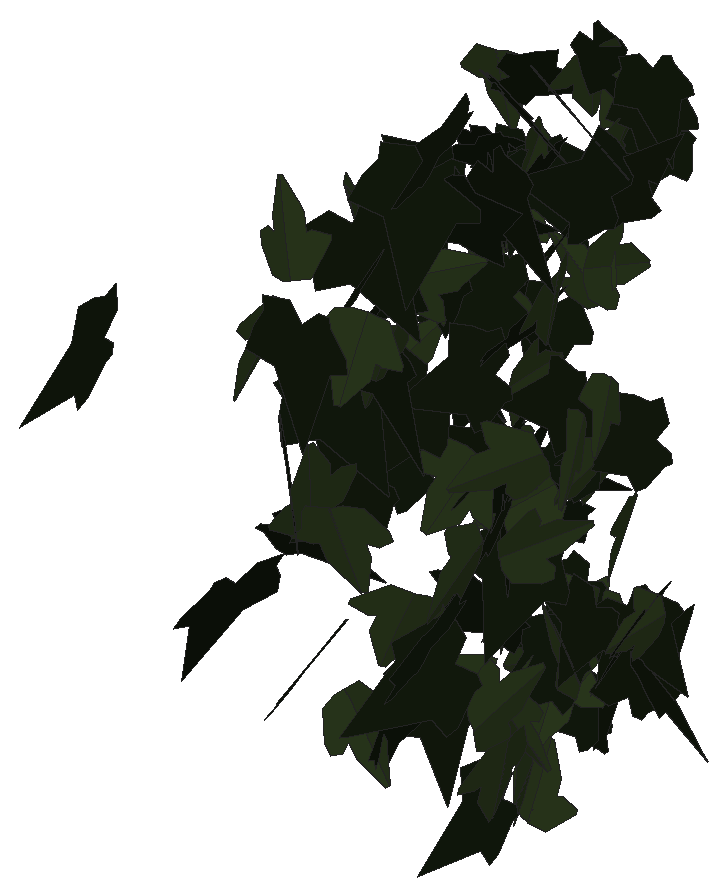
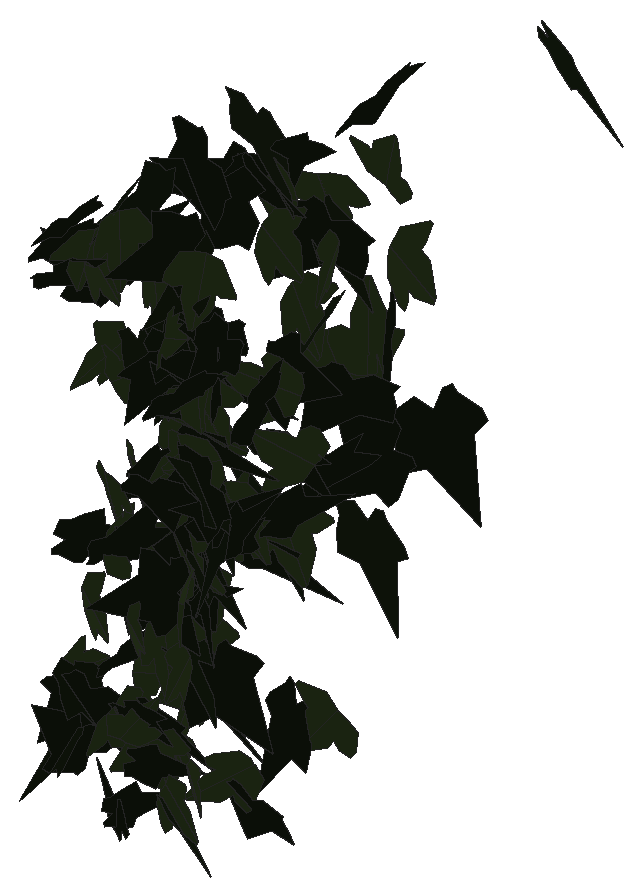
# SketchUp Ruby script. Lengths in inches.
U = 1.inch
M = Sketchup.active_model
def pt(a) = Geom::Point3d.new(a.map { |v| v * U })
def face(e, loops, mat)
  f = e.add_face(loops[0].map { |a| pt(a) })
  loops[1..].each { |l| e.add_face(l.map { |a| pt(a) }).erase! }
  f.material = f.back_material = mat if mat
  f
end
# faces: each face lists its corners as indices into pts; further lists are holes
def faces(e, pts, list, mat = nil) = list.each { |f| face(e, (f[0].is_a?(Array) ? f : [f]).map { |l| l.map { |i| pts[i] } }, mat) }
# xy, xz, yz: faces in a plane at the given z, y or x. An outline is a flat list of corners, or four numbers for a rectangle; further outlines are holes
def ring(l) = l.size == 4 ? [[l[0], l[1]], [l[2], l[1]], [l[2], l[3]], [l[0], l[3]]] : l.each_slice(2).to_a
def flat(e, list, mat, &to3) = list.each { |f| face(e, (f[0].is_a?(Array) ? f : [f]).map { |l| ring(l).map { |u, v| to3.(u, v) } }, mat) }
def xy(e, z, list, mat = nil) = flat(e, list, mat) { |x, y| [x, y, z] }
def xz(e, y, list, mat = nil) = flat(e, list, mat) { |x, z| [x, y, z] }
def yz(e, x, list, mat = nil) = flat(e, list, mat) { |y, z| [x, y, z] }
def lines(e, pts, list) = list.each { |a, b| e.add_line(pt(pts[a]), pt(pts[b])) }
# prism: a flat outline (further loops are holes) pulled along v
def prism(e, loops, v, mat = nil)
  f = face(e, loops, mat); d = Geom::Vector3d.new(v.map { |x| x * U })
  f.pushpull(f.normal.samedirection?(d) ? d.length : -d.length)
end
def box(e, o, s, mat = nil) = prism(e, [[o, [o[0] + s[0], o[1], o[2]], [o[0] + s[0], o[1] + s[1], o[2]], [o[0], o[1] + s[1], o[2]]]], [0, 0, s[2]], mat)
def at(x, y, z, deg = 0) = Geom::Transformation.translation(pt([x, y, z])) * Geom::Transformation.rotation(ORIGIN, Z_AXIS, deg.degrees)
def axes(o, x, y, z) = Geom::Transformation.new([*x, 0, *y, 0, *z, 0, *pt(o).to_a, 1])
def part(name) = M.definitions.add(name)
# library, detail: a bought-in or finely detailed component or shape, given as its bounding box
def library(name, o, s) = part(name).tap { |d| box(d.entities, o, s) }
def detail(e, o, s) = box(e.add_group.entities, o, s)
def put(e, d, t, mat = nil) = e.add_instance(d, t).tap { |i| i.material = mat if mat }
def group(e, t, mat = nil) = e.add_group.tap { |g| g.transformation = t; g.material = mat if mat }.entities
root = M.entities
M.materials.add("efeu1").color = [18, 25, 13]
M.materials.add("efeu2").color = [43, 57, 29]
c1 = part("ivyleaf_9")
p = [[1.54,2.16,1.25],[1.36,2.04,1.19],[-0.21,0.99,0.68],[-0.71,1.11,0.82],[-0.85,0.86,0.67],[-0.8,0.17,0.21],
  [-0.9,-0.01,0.1],[-0.67,-0.16,-0.02],[-0.08,-0.08,-0.05],[-0.03,-0.6,-0.4],[0.65,-0.88,-0.66],[0.83,-0.6,-0.49],
  [1.29,-0.42,-0.43],[1.8125,-0.07,-0.26],[1.21,0.44,0.15]]
faces(c1.entities,p,[[0,1,2,3,4,5,6,7,8,9,10,11,12,13,14]],"efeu1")
c2 = part("ivyleaf_10")
p = [[0,0.5,-0.03],[-0.0625,2.02,-0.43],[-0.19,2.01,-0.46],[-0.54,1.05,-0.29],[-0.52,0.625,-0.18],[-0.83,0.76,-0.28],
  [-1.16,0.64,-0.33],[-1.15,0.33,-0.24],[-0.77,-0.39,0.02],[-0.3,-0.51,0.16],[0.04,-0.48,0.23],[-0.02,2.01,-0.4375],
  [-0.06,2.01,-0.43],[0.04,-0.49,0.23],[0.67,-0.49,0.14],[1.38,0.36,-0.2],[1.375,0.51,-0.24],[0.81,0.65,-0.19],
  [0.62,0.59,-0.15],[0.6,1.09,-0.28],[0.5,1.23,-0.31]]
faces(c2.entities,p,[[0,1,2,3,4,5,6,7,8,9,10],[11,12,0,13,14,15,16,17,18,19,20]],"efeu2")
put(root,c1,axes([594.9,111.1,205.24],[-1.20311,0.67443,-0.22377],[0.18999,-0.11868,-1.37921],[-0.68471,-1.21797,0.01049]))
put(root,c1,axes([598.09,116.25,204.45],[0.0745,-1.25549,0.12259],[0.01675,-0.12181,-1.25766],[1.26135,0.07578,0.00946]))
put(root,c1,axes([594.7,117.4375,194.38],[-0.30601,1.14013,-0.69859],[0.15547,-0.68145,-1.18026],[-1.32807,-0.34248,0.0228]))
put(root,c2,axes([596.25,119.11,196.8125],[-0.28548,-1.16466,-0.34594],[-0.08339,-0.33574,1.19914],[-1.21208,0.29741,-0.00102]))
put(root,c1,axes([594.87,119.52,197.96],[0.12828,-0.08477,-1.23247],[1.18885,-0.3284,0.14633],[-0.33586,-1.19482,0.04722]))
put(root,c2,axes([597.12,119.09,196.59],[-1.14088,-0.33532,-0.23766],[0.23576,0.04044,-1.18883],[0.33666,-1.16467,0.02715]))
put(root,c2,axes([597.57,119.52,202.76],[1.09698,0.24304,-0.16363],[-0.15952,-0.03646,-1.12358],[-0.24576,1.10852,-0.00108]))
put(root,c2,axes([593.89,120.15,201.63],[0.2666,-0.99216,0.69498],[0.16277,-0.67582,-1.02724],[1.20037,0.312,-0.01506]))
put(root,c2,axes([594.92,119.72,204.11],[1.07624,-0.08575,0.44382],[-0.43931,0.07148,1.07913],[-0.10645,-1.16196,0.03363]))
put(root,c1,axes([595.5,119.875,191.06],[-0.49456,1.21146,0.07928],[-0.03156,0.07275,-1.30852],[-1.21364,-0.49556,0.00172]))
put(root,c1,axes([594.05,120.63,194.66],[1.08809,0.26212,0.32005],[0.31075,0.0766,-1.11922],[-0.27308,1.1316,0.00162]))
put(root,c1,axes([596.14,121.25,202.8],[-0.74032,0.84807,-0.33833],[0.22298,-0.25445,-1.12574],[-0.88542,-0.77317,-0.00062]))
put(root,c1,axes([598.46,121.56,191.92],[-0.60702,1.1525,0.22615],[-0.15966,0.17124,-1.30117],[-1.16357,-0.62474,0.06056]))
put(root,c1,axes([598.18,122.84,190.66],[-1.26764,-0.15024,0.27481],[-0.26251,-0.11522,-1.27389],[0.17082,-1.29195,0.08166]))
put(root,c2,axes([596.03,122.76,200.54],[-0.0207,-1.07947,0.24208],[-0.01252,-0.24187,-1.07964],[1.1062,-0.02294,-0.00769]))
put(root,c2,axes([596.7,122.82,192.1],[-0.77403,-0.71989,0.40358],[-0.28667,-0.28432,-1.05698],[0.77391,-0.82532,0.01211]))
put(root,c1,axes([594.84,122.74,203.73],[-0.33428,-0.44901,-1.13368],[0.79121,0.81456,-0.55592],[0.9278,-0.85642,0.06562]))
put(root,c1,axes([596.86,123.4375,205.82],[-0.50897,-1.17452,-0.21721],[0.05931,0.21096,-1.27973],[1.19297,-0.51159,-0.02905]))
put(root,c1,axes([594.5,123.87,194.94],[-0.45546,-0.7442,0.79182],[-0.36336,-0.70483,-0.87145],[1.0241,-0.58106,0.04295]))
put(root,c1,axes([593.81,122.88,198.29],[-0.2402,-0.7174,-0.98343],[0.52576,0.84293,-0.74333],[1.09789,-0.56061,0.14081]))
put(root,c1,axes([595.05,123.26,199.78],[0.70864,-1.15375,-0.04659],[-0.01528,0.04529,-1.35395],[1.15458,0.70872,0.01068]))
put(root,c1,axes([597.48,123.1,206.84],[-0.53357,1.12789,0.44328],[-0.27597,0.35853,-1.24444],[-1.18003,-0.59384,0.09059]))
put(root,c2,axes([595.58,124.06,204.99],[-0.32373,0.31033,-1.05872],[0.8146,-0.67688,-0.44749],[-0.74406,-0.87608,-0.02929]))
put(root,c2,axes([599.0625,124.15,187.55],[0.00145,-1.23722,-0.02442],[0.0218,0.02444,-1.23703],[1.23727,0.00102,0.02182]))
put(root,c2,axes([597.16,124.94,192.93],[0.12007,-0.39198,1.14556],[0.44623,-1.05582,-0.40804],[1.12554,0.4604,0.03957]))
put(root,c1,axes([596.91,123.91,205.14],[-0.72385,-0.02588,-0.87365],[-0.87227,-0.05072,0.72421],[-0.05556,1.13343,0.01246]))
put(root,c2,axes([593.65,124.12,203.65],[-0.7185,0.75396,-0.07109],[0.04465,-0.05565,-1.04148],[-0.75599,-0.71987,0.00605]))
put(root,c1,axes([598.65,124.46,185.74],[-1.17691,0.31113,-0.06093],[0.05753,-0.0208,-1.21733],[-0.31177,-1.1783,0.0054]))
put(root,c1,axes([597.14,124.28,204.4375],[0.75648,0.33779,-0.92743],[0.76873,0.53128,0.82054],[0.6191,-1.07244,0.11438]))
put(root,c2,axes([593.26,124.52,186.78],[0.85944,0.05689,0.79181],[0.78275,0.13373,-0.85922],[-0.13229,1.16091,0.06018]))
put(root,c1,axes([598.35,124.74,205.71],[-0.18682,-0.06636,-1.28296],[1.23249,0.35651,-0.19791],[0.36245,-1.24651,0.01169]))
put(root,c2,axes([598.74,123.77,188.82],[0.07731,0.27266,-1.16452],[0.37166,1.1037,0.28309],[1.13681,-0.37938,-0.01336]))
put(root,c2,axes([594.9,125.6,204.46],[0.07768,-0.94291,0.60554],[0.09727,-0.59903,-0.94525],[1.11638,0.1178,0.04023]))
put(root,c2,axes([598.57,125.69,196.26],[-0.2748,-0.36508,1.04422],[-0.64122,-0.82417,-0.45689],[0.90139,-0.69759,-0.00668]))
put(root,c1,axes([594.84,125.72,197],[-1.18345,-0.33009,-0.14086],[0.14235,0.01385,-1.22838],[0.32945,-1.19173,0.02474]))
put(root,c1,axes([597.35,125.73,198.55],[-0.96344,0.00137,0.49421],[-0.49418,0.00887,-0.96341],[-0.00527,-1.08276,-0.00727]))
put(root,c1,axes([594.375,126.14,194.43],[-0.43172,-0.27867,0.83565],[-0.63499,-0.54656,-0.51031],[0.61054,-0.76549,0.06015]))
put(root,c1,axes([594.01,126.54,200.28],[-0.50797,0.10068,-0.93521],[0.47648,-0.88887,-0.3545],[-0.81101,-0.58529,0.3775]))
put(root,c1,axes([594.47,124.98,186.88],[-0.14259,0.12416,-1.22895],[-0.85525,0.88268,0.18841],[0.89122,0.86691,-0.01583]))
put(root,c2,axes([597.86,126.67,185.43],[-0.04899,0.07828,1.13161],[0.76419,-0.83476,0.09083],[0.83826,0.76558,-0.01667]))
put(root,c2,axes([596,126.24,194.73],[1.11903,-0.15908,-0.48461],[-0.4793,0.07159,-1.13028],[0.17442,1.21736,0.00314]))
put(root,c2,axes([599.24,126.19,201.95],[0.22876,-1.14299,-0.23813],[-0.03512,0.23581,-1.1656],[1.167,0.23115,0.0116]))
put(root,c2,axes([597.5,126.34,187.57],[-0.71977,0.24817,-0.71613],[0.66548,-0.26573,-0.76094],[-0.36273,-0.97995,0.02498]))
put(root,c2,axes([593.23,126.08,197.03],[0.47905,0.46185,-0.89118],[0.64311,0.61694,0.66542],[0.77066,-0.80192,-0.00133]))
put(root,c2,axes([598.19,126.7,184.47],[1.00415,-0.13155,-0.12814],[0.12988,0.00515,1.0125],[-0.12983,-1.01228,0.0218]))
put(root,c1,axes([596.81,126.48,195.22],[-0.41451,1.0853,0.27622],[-0.14478,0.24013,-1.16076],[-1.1105,-0.4364,0.04823]))
put(root,c1,axes([597.64,126.23,199.7],[0.25674,0.98822,0.60672],[0.05834,0.60962,-1.01763],[-1.15814,0.24978,0.08324]))
put(root,c1,axes([596.46,127.47,193.17],[-0.85719,0.52427,-0.63273],[0.52037,-0.36129,-1.00433],[-0.63594,-1.00229,0.03106]))
put(root,c2,axes([593.42,126.91,199.89],[0.33092,0.06052,-1.1124],[1.08765,0.23357,0.33627],[0.24108,-1.13683,0.00987]))
put(root,c2,axes([597.75,126.57,192.53],[0.07707,-0.32794,1.07701],[0.26087,1.05535,0.30268],[-1.09519,0.22831,0.14789]))
put(root,c1,axes([595.4,127.75,194.13],[0.13124,0.00441,0.93921],[-0.90052,-0.26881,0.1271],[0.26681,-0.90944,-0.03301]))
put(root,c1,axes([593.59,128.3,199.82],[0.23887,-0.51465,-1.0461],[0.55581,-0.88839,0.56399],[-1.02482,-0.60177,0.06204]))
put(root,c1,axes([596.72,128.18,191.48],[-0.58311,-1.01327,0.05954],[0.0237,-0.08224,-1.16746],[1.01475,-0.58034,0.06148]))
put(root,c1,axes([596.42,127.47,192.54],[0.1951,-0.0134,-1.18093],[-1.17095,0.15371,-0.19519],[0.15383,1.18703,0.01194]))
put(root,c2,axes([598.39,128.28,195.9],[0.88414,-0.70101,0.1802],[0.14546,-0.10659,-1.1283],[0.70904,0.896,0.00677]))
put(root,c1,axes([599.05,128.9,203.59],[-0.13514,-0.10869,1.14619],[-0.86731,-0.74937,-0.17332],[0.75719,-0.87776,0.00605]))
put(root,c2,axes([596.95,128.33,193.45],[0.73138,0.04132,-0.84086],[-0.83782,-0.07346,-0.73235],[-0.08253,1.11201,-0.01714]))
put(root,c1,axes([595.26,128.1,189.43],[0.06919,0.53824,-1.02259],[-0.86814,-0.65192,-0.40188],[-0.7627,0.79087,0.36467]))
put(root,c1,axes([593.3,128.62,185.47],[-0.60254,-0.44485,-0.79269],[0.79197,0.20986,-0.71976],[0.44614,-0.97333,0.20711]))
put(root,c1,axes([596.26,127.46,193.14],[0.08916,0.08245,1.19053],[0.4124,1.11817,-0.10832],[-1.11986,0.41834,0.05489]))
put(root,c1,axes([596.62,127.98,190.29],[-0.5249,1.0271,0.21942],[-0.11604,0.18708,-1.15332],[-1.04385,-0.53727,0.01787]))
put(root,c1,axes([597.55,129.27,196.27],[0.05233,-0.73378,-0.62109],[0.15857,-0.60691,0.73038],[-0.94818,-0.14199,0.08786]))
put(root,c2,axes([598.28,128.1,188.27],[-0.30993,0.35557,-0.99241],[-0.70903,0.69518,0.47051],[0.78013,0.77309,0.03336]))
put(root,c1,axes([598.16,129.4,189.58],[-0.24689,-0.83209,0.37404],[-0.06986,-0.36911,-0.86724],[0.90962,-0.25419,0.03491]))
put(root,c1,axes([593.74,129.49,195.25],[-0.12385,-0.18483,0.88129],[-0.48049,-0.73878,-0.22247],[0.76155,-0.49619,0.00296]))
put(root,c2,axes([593.94,128.44,186.23],[-0.39005,-0.289,-0.83354],[0.74463,0.38091,-0.48051],[0.47312,-0.83776,0.06907]))
put(root,c1,axes([597.03,128.96,206.24],[0.91232,-0.61368,0.33504],[0.29202,-0.16602,-1.09925],[0.63529,0.95761,0.02413]))
put(root,c2,axes([595.38,129.4375,193.61],[-0.03839,-0.0636,-0.9919],[0.66321,-0.74099,0.02184],[-0.74031,-0.66051,0.071]))
put(root,c1,axes([597.15,129.39,187.81],[-1.1226,0.03762,0.0796],[-0.08039,-0.02268,-1.12295],[-0.03591,-1.12519,0.0253]))
put(root,c2,axes([596.39,128.38,196.81],[0.08525,-0.0547,0.92635],[-0.24421,0.89614,0.07539],[-0.89525,-0.24966,0.06764]))
put(root,c1,axes([596.7,129.43,192.39],[0.08789,0.45969,-0.76832],[-0.18811,-0.7453,-0.46744],[-0.87535,0.20631,0.02331]))
put(root,c1,axes([594.95,129.56,198.56],[-0.8881,0.06353,0.49285],[-0.49544,-0.035,-0.88825],[-0.0385,-1.01509,0.06147]))
put(root,c2,axes([597.7,130.18,194.02],[-0.00668,-0.17973,1.03263],[0.27265,-0.9974,-0.17184],[1.01208,0.26751,0.0531]))
put(root,c2,axes([596.57,129.72,186.79],[0.73709,0.75243,-0.3262],[-0.20901,-0.25176,-1.05299],[-0.79302,0.76572,-0.02566]))
put(root,c2,axes([596.04,129.65,191.29],[-0.18669,-1.12325,-0.10035],[0.02217,0.09804,-1.13865],[1.12751,-0.18791,0.00577]))
put(root,c1,axes([598.72,129.3,203.11],[-0.19393,-0.11076,1.00396],[0.99024,0.18065,0.21121],[-0.19909,1.00643,0.07258]))
put(root,c2,axes([597.92,129.7,199.92],[0.58175,0.12471,0.73637],[-0.71828,-0.16232,0.59494],[0.20463,-0.9243,-0.00512]))
put(root,c1,axes([593.91,129.375,203.18],[0.46316,0.63616,-0.0337],[-0.02211,-0.02559,-0.78689],[-0.63666,0.46368,0.00281]))
put(root,c1,axes([594.5,129.64,205.19],[1.0217,-0.22836,-0.10217],[-0.0933,0.05079,-1.0465],[0.23212,1.02554,0.02908]))
put(root,c2,axes([598,130.08,196.27],[0.84289,-0.38723,0.13799],[0.12628,-0.05566,-0.92758],[0.3912,0.8523,0.00212]))
put(root,c1,axes([597.1,129.74,201.58],[-0.46856,0.78495,-0.04748],[0.02095,-0.04278,-0.91416],[-0.78611,-0.46901,0.00394]))
put(root,c1,axes([593.45,130.33,202.03],[-0.01983,0.00992,-0.97393],[0.96818,-0.10596,-0.02079],[-0.10614,-0.96835,-0.0077]))
put(root,c2,axes([599.17,130.7,189.02],[-0.00874,-0.04692,0.92251],[0.15898,-0.90886,-0.04472],[0.90992,0.15834,0.01667]))
put(root,c2,axes([598.25,130.48,204.6],[0.23825,-0.90245,0.42845],[0.11251,-0.41342,-0.93336],[0.99263,0.26347,0.00296]))
put(root,c2,axes([593.99,130.08,198.4],[-0.46192,0.07919,-0.839],[0.82019,-0.17754,-0.46832],[-0.19359,-0.94115,0.01775]))
put(root,c1,axes([593.65,129.72,195.66],[0.62204,-0.1453,-0.68342],[-0.63983,0.24916,-0.63534],[0.28071,0.8899,0.0663]))
put(root,c2,axes([598.4375,129.33,200.8],[-0.04992,0.28687,1.01127],[-0.15941,0.99864,-0.29116],[-1.03902,-0.167,-0.00391]))
put(root,c1,axes([597.63,130.26,193.91],[-0.64389,-0.92695,0.25572],[0.14532,0.21041,1.12864],[-0.95053,0.66008,-0.00067]))
put(root,c1,axes([595.46,130.42,202.73],[-0.45107,0.60726,-0.57818],[0.3163,-0.48479,-0.75594],[-0.77654,-0.5502,0.02794]))
put(root,c2,axes([594.13,130.43,200.99],[0.92449,0.48477,-0.38729],[-0.34046,-0.18468,-1.04387],[-0.51874,0.98517,-0.00511]))
put(root,c1,axes([595.04,129.68,205.7],[0.6894,0.31815,0.61576],[0.57362,0.22558,-0.75877],[-0.38903,0.8964,-0.0276]))
put(root,c2,axes([594.15,130.22,205.56],[-1.04587,-0.14242,-0.04362],[0.05388,-0.07332,-1.05249],[0.13886,-1.04421,0.07985]))
put(root,c1,axes([593.35,129.98,203.08],[0.75165,0.19862,-0.06725],[-0.06261,-0.02628,-0.7774],[-0.20013,0.7542,-0.00938]))
put(root,c2,axes([594.99,130.9,203.06],[-0.05005,0.49555,-0.81179],[0.01512,-0.81239,-0.49685],[-0.95097,-0.039,0.03482]))
put(root,c1,axes([595.5,129.95,192.99],[0.73936,0.13135,0.63669],[0.62316,0.13147,-0.75078],[-0.18518,0.96682,0.0156]))
put(root,c2,axes([598.25,130.82,192.2],[0.44722,-0.80603,0.40219],[0.19143,-0.35374,-0.92178],[0.88022,0.48645,-0.00388]))
put(root,c1,axes([593.69,129.91,197.125],[-0.28008,0.92287,-0.00056],[-0.00182,0.00003,0.96443],[0.92287,0.28008,0.00173]))
put(root,c1,axes([599.02,130.57,189.2],[-0.60864,0.75542,-0.5157],[0.28673,-0.43064,-0.96922],[-0.86855,-0.67153,0.04141]))
put(root,c2,axes([593.93,130.67,201.36],[0.40864,0.86846,-0.1499],[-0.05932,-0.13775,-0.95978],[-0.8793,0.41289,-0.00491]))
put(root,c1,axes([593.52,130.68,198],[-0.01278,0.0045,-1.1103],[1.02187,0.43433,-0.01],[0.43426,-1.02191,-0.00914]))
put(root,c1,axes([598.71,131.31,194.45],[-0.56689,-0.33915,0.724],[-0.62907,-0.35855,-0.66051],[0.49343,-0.84675,-0.0103]))
put(root,c2,axes([596.98,131.05,188.49],[0.14125,0.94566,-0.59477],[-0.11135,-0.5846,-0.95594],[-1.11159,0.17872,0.02018]))
put(root,c2,axes([594.53,130.7,190.99],[-0.66548,0.50109,-0.25611],[0.20931,-0.14777,-0.83301],[-0.52237,-0.69758,-0.00751]))
put(root,c1,axes([596.8125,131.29,185],[-0.34639,-0.20912,0.70477],[-0.56676,-0.42023,-0.40325],[0.4682,-0.6634,0.03328]))
put(root,c1,axes([597.1875,130.71,207],[0.65166,-0.72239,-0.34968],[-0.16409,0.321,-0.96893],[0.78562,0.66626,0.08768]))
put(root,c1,axes([595.95,131.2,187.14],[-0.22726,-0.31106,-0.66137],[-0.4042,-0.52355,0.38513],[-0.60892,0.46362,-0.00881]))
put(root,c2,axes([596.96,130.87,206.39],[-0.29812,-0.9845,-0.10293],[0.04545,0.09377,-1.02852],[0.98883,-0.30113,0.01625]))
put(root,c1,axes([595.26,131.23,197.6],[-0.72958,-0.54805,-0.39857],[0.35621,0.18806,-0.91063],[0.57649,-0.8098,0.05826]))
put(root,c1,axes([594.86,130.6875,185.32],[-0.52266,0.60055,0.31657],[-0.21118,0.23588,-0.79612],[-0.6452,-0.56369,0.00413]))
put(root,c1,axes([596.3125,131.29,189],[-0.74256,-0.23828,-0.01018],[0.01007,0.00193,-0.77986],[0.23829,-0.74263,0.00124]))
put(root,c1,axes([599.01,131.62,204.375],[-0.60396,-0.68215,0.21429],[-0.06116,-0.2302,-0.90515],[0.7124,-0.59808,0.10397]))
put(root,c2,axes([593.81,131.11,187.3],[0.36988,-0.60375,-0.00174],[-0.00087,0.0015,-0.70804],[0.60375,0.36988,0.00004]))
put(root,c1,axes([598.87,131.41,205.59],[-0.19605,-0.91452,-0.13606],[0.02971,0.13278,-0.9353],[0.92411,-0.19829,0.00121]))
put(root,c1,axes([596.66,131.29,184.53],[-0.10799,0.2795,0.74892],[0.32028,-0.67729,0.29895],[0.73241,0.33738,-0.0203]))
put(root,c2,axes([596.33,131.24,188.1],[0.38044,0.54273,0.41708],[-0.23579,-0.34406,0.66278],[0.64259,-0.44757,-0.00374]))
put(root,c2,axes([594.84,130.96,186.09],[-0.40561,0.08531,0.80091],[-0.80136,0.04734,-0.41088],[-0.08091,-0.89651,0.05451]))
put(root,c1,axes([598.71,131.38,206.36],[0.11162,-0.92575,-0.17275],[0.0434,0.17883,-0.93029],[0.94073,0.10159,0.06342]))
put(root,c2,axes([594.64,130.55,193.19],[-0.15484,0.42908,-0.88912],[-0.38922,0.80056,0.45412],[0.90728,0.41667,0.04308]))
put(root,c1,axes([598.74,131,187.28],[0.94308,-0.57897,-0.34694],[-0.27663,0.21221,-1.10608],[0.61567,0.98221,0.03446]))
put(root,c1,axes([598.17,131.03,188.88],[-0.23891,-0.3734,-0.91187],[0.4917,0.76795,-0.44329],[0.85392,-0.54667,0.00013]))
put(root,c1,axes([598.48,130.68,186.45],[-0.28334,-0.18318,0.99106],[0.85342,0.50402,0.33715],[-0.53612,0.89913,0.01291]))
put(root,c1,axes([594.92,131.11,202.24],[-0.01985,-0.73608,-0.71535],[0.07072,0.7128,-0.73542],[1.02398,-0.0635,0.03692]))
put(root,c2,axes([597.97,131.11,205.73],[0.25548,0.99358,0.11453],[0.04438,0.10683,-1.02577],[-0.99917,0.2588,-0.01628]))
put(root,c1,axes([593.87,131.83,201.78],[-0.25088,-0.99837,0.03488],[-0.01168,-0.03302,-1.0294],[0.99891,-0.25113,-0.00328]))
put(root,c2,axes([595.85,131.63,192.41],[0.37949,-0.53965,0.38028],[0.21926,-0.31071,-0.65972],[0.62271,0.43827,0.00054]))
